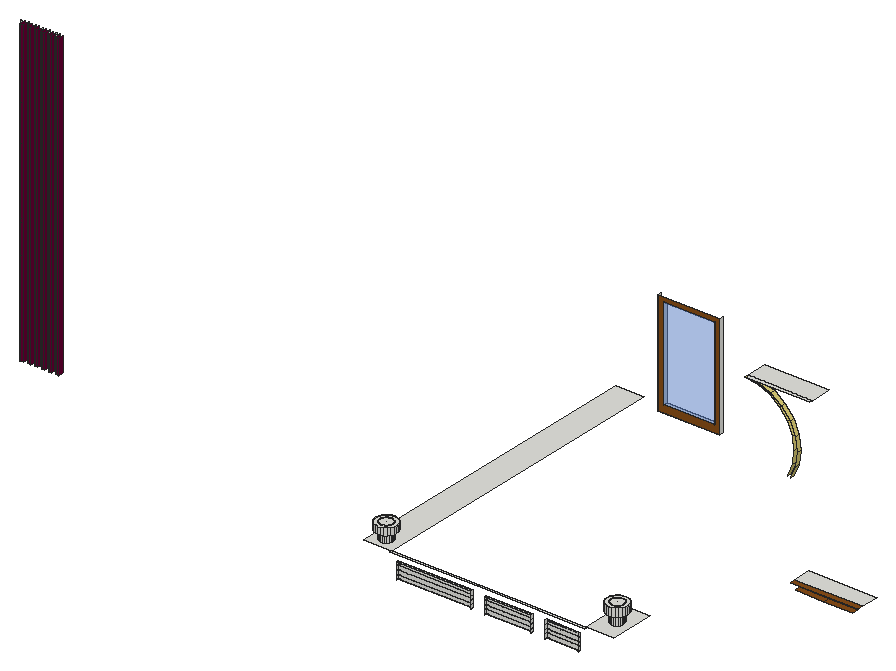
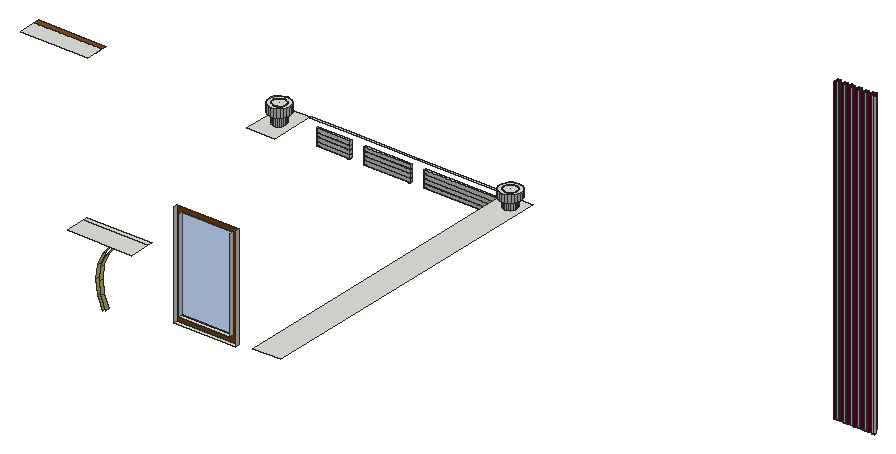
# SketchUp Ruby script. Lengths in inches.
U = 1.inch
M = Sketchup.active_model
def pt(a) = Geom::Point3d.new(a.map { |v| v * U })
def face(e, loops, mat)
  f = e.add_face(loops[0].map { |a| pt(a) })
  loops[1..].each { |l| e.add_face(l.map { |a| pt(a) }).erase! }
  f.material = f.back_material = mat if mat
  f
end
# faces: each face lists its corners as indices into pts; further lists are holes
def faces(e, pts, list, mat = nil) = list.each { |f| face(e, (f[0].is_a?(Array) ? f : [f]).map { |l| l.map { |i| pts[i] } }, mat) }
# xy, xz, yz: faces in a plane at the given z, y or x. An outline is a flat list of corners, or four numbers for a rectangle; further outlines are holes
def ring(l) = l.size == 4 ? [[l[0], l[1]], [l[2], l[1]], [l[2], l[3]], [l[0], l[3]]] : l.each_slice(2).to_a
def flat(e, list, mat, &to3) = list.each { |f| face(e, (f[0].is_a?(Array) ? f : [f]).map { |l| ring(l).map { |u, v| to3.(u, v) } }, mat) }
def xy(e, z, list, mat = nil) = flat(e, list, mat) { |x, y| [x, y, z] }
def xz(e, y, list, mat = nil) = flat(e, list, mat) { |x, z| [x, y, z] }
def yz(e, x, list, mat = nil) = flat(e, list, mat) { |y, z| [x, y, z] }
def lines(e, pts, list) = list.each { |a, b| e.add_line(pt(pts[a]), pt(pts[b])) }
# prism: a flat outline (further loops are holes) pulled along v
def prism(e, loops, v, mat = nil)
  f = face(e, loops, mat); d = Geom::Vector3d.new(v.map { |x| x * U })
  f.pushpull(f.normal.samedirection?(d) ? d.length : -d.length)
end
def box(e, o, s, mat = nil) = prism(e, [[o, [o[0] + s[0], o[1], o[2]], [o[0] + s[0], o[1] + s[1], o[2]], [o[0], o[1] + s[1], o[2]]]], [0, 0, s[2]], mat)
def at(x, y, z, deg = 0) = Geom::Transformation.translation(pt([x, y, z])) * Geom::Transformation.rotation(ORIGIN, Z_AXIS, deg.degrees)
def axes(o, x, y, z) = Geom::Transformation.new([*x, 0, *y, 0, *z, 0, *pt(o).to_a, 1])
def part(name) = M.definitions.add(name)
# library, detail: a bought-in or finely detailed component or shape, given as its bounding box
def library(name, o, s) = part(name).tap { |d| box(d.entities, o, s) }
def detail(e, o, s) = box(e.add_group.entities, o, s)
def put(e, d, t, mat = nil) = e.add_instance(d, t).tap { |i| i.material = mat if mat }
def group(e, t, mat = nil) = e.add_group.tap { |g| g.transformation = t; g.material = mat if mat }.entities
root = M.entities
M.materials.add("Teddy_SkinShadow ").color = [134, 77, 23]
M.materials.add("[Color L16]").color = [102, 0, 51]
M.materials.add("[Translucent Glass Blue]").color = [100, 149, 237]
M.materials["[Translucent Glass Blue]"].alpha = 0.5
M.materials.add("[Wood Board Cork]").color = [215, 201, 115]
xy(root,49.297,[[880.196,111.916,881.943,112.729],[883.778,111.916,885.525,112.729],[887.36,111.916,889.107,112.729],[869.45,112.041,871.197,112.729],[873.032,112.041,874.779,112.729],
  [876.614,112.041,878.361,112.729]])
xy(root,49.297,[[871.241,109.541,872.988,112.729],[881.987,109.854,883.734,112.729],[885.569,109.854,887.316,112.729],[889.151,109.854,890.942,112.729],[874.823,109.979,876.57,112.729],
  [878.405,109.979,880.152,112.729]],"[Color L16]")
xy(root,56.441,[[1147.452,64.973,1171.711,65.973],[1178.83,64.973,1196.125,65.973]])
xy(root,56.645,[[1101.817,64.973,1140.537,65.973]])
xy(root,57.564,[[1107.504,227.266,1139.629,229.266]])
xy(root,60,[[1098.461,64.973,1143.893,65.973],[1143.893,64.973,1175.271,65.973],[1175.271,64.973,1199.684,65.973],[[1084.247,65.973,1098.461,229.266],[1090.628,69,1089.738,69.117,1088.909,69.461,1088.197,70.007,1087.651,70.719,1087.308,71.548,1087.19,72.4375,1087.308,73.327,1087.651,74.156,1088.197,74.868,1088.909,75.414,1089.738,75.758,1090.628,75.875,1091.518,75.758,1092.347,75.414,1093.059,74.868,1093.605,74.156,1093.948,73.327,1094.065,72.4375,1093.948,71.548,1093.605,70.719,1093.059,70.007,1092.347,69.461,1091.518,69.117]]])
xy(root,60.1875,[[[1199.684,65.973,1213.899,88.973],[1206.602,73.728,1205.713,73.845,1204.883,74.189,1204.172,74.735,1203.625,75.447,1203.282,76.276,1203.165,77.166,1203.282,78.055,1203.625,78.884,1204.172,79.596,1204.883,80.143,1205.713,80.486,1206.602,80.603,1207.492,80.486,1208.321,80.143,1209.033,79.596,1209.579,78.884,1209.923,78.055,1210.04,77.166,1209.923,76.276,1209.579,75.447,1209.033,74.735,1208.321,74.189,1207.492,73.845]]])
xy(root,61.264,[[1110.481,227.266,1136.918,229.266]])
xy(root,64.5,[[[1090.628,66.975,1089.214,67.161,1087.897,67.707,1086.765,68.575,1085.897,69.706,1085.352,71.024,1085.165,72.4375,1085.352,73.851,1085.897,75.169,1086.765,76.3,1087.897,77.168,1089.214,77.714,1090.628,77.9,1092.042,77.714,1093.359,77.168,1094.491,76.3,1095.359,75.169,1095.904,73.851,1096.091,72.4375,1095.904,71.024,1095.359,69.706,1094.491,68.575,1093.359,67.707,1092.042,67.161],[1090.628,69,1091.518,69.117,1092.347,69.461,1093.059,70.007,1093.605,70.719,1093.948,71.548,1094.065,72.4375,1093.948,73.327,1093.605,74.156,1093.059,74.868,1092.347,75.414,1091.518,75.758,1090.628,75.875,1089.738,75.758,1088.909,75.414,1088.197,74.868,1087.651,74.156,1087.308,73.327,1087.19,72.4375,1087.308,71.548,1087.651,70.719,1088.197,70.007,1088.909,69.461,1089.738,69.117]]])
xy(root,65.375,[[[1206.602,71.703,1205.188,71.889,1203.871,72.435,1202.74,73.303,1201.871,74.434,1201.326,75.752,1201.14,77.166,1201.326,78.579,1201.871,79.897,1202.74,81.028,1203.871,81.896,1205.188,82.442,1206.602,82.628,1208.016,82.442,1209.333,81.896,1210.465,81.028,1211.333,79.897,1211.879,78.579,1212.065,77.166,1211.879,75.752,1211.333,74.434,1210.465,73.303,1209.333,72.435,1208.016,71.889],[1206.602,73.728,1207.492,73.845,1208.321,74.189,1209.033,74.735,1209.579,75.447,1209.923,76.276,1210.04,77.166,1209.923,78.055,1209.579,78.884,1209.033,79.596,1208.321,80.143,1207.492,80.486,1206.602,80.603,1205.713,80.486,1204.883,80.143,1204.172,79.596,1203.625,78.884,1203.282,78.055,1203.165,77.166,1203.282,76.276,1203.625,75.447,1204.172,74.735,1204.883,74.189,1205.713,73.845]]])
xy(root,68.125,[[[1090.628,66.975,1092.042,67.161,1093.359,67.707,1094.491,68.575,1095.359,69.706,1095.904,71.024,1096.091,72.4375,1095.904,73.851,1095.359,75.169,1094.491,76.3,1093.359,77.168,1092.042,77.714,1090.628,77.9,1089.214,77.714,1087.897,77.168,1086.765,76.3,1085.897,75.169,1085.352,73.851,1085.165,72.4375,1085.352,71.024,1085.897,69.706,1086.765,68.575,1087.897,67.707,1089.214,67.161],[1090.628,69,1089.738,69.117,1088.909,69.461,1088.197,70.007,1087.651,70.719,1087.308,71.548,1087.19,72.4375,1087.308,73.327,1087.651,74.156,1088.197,74.868,1088.909,75.414,1089.738,75.758,1090.628,75.875,1091.518,75.758,1092.347,75.414,1093.059,74.868,1093.605,74.156,1093.948,73.327,1094.065,72.4375,1093.948,71.548,1093.605,70.719,1093.059,70.007,1092.347,69.461,1091.518,69.117]],[1090.628,69,1091.518,69.117,1092.347,69.461,1093.059,70.007,1093.605,70.719,1093.948,71.548,1094.065,72.4375,1093.948,73.327,1093.605,74.156,1093.059,74.868,1092.347,75.414,1091.518,75.758,1090.628,75.875,1089.738,75.758,1088.909,75.414,1088.197,74.868,1087.651,74.156,1087.308,73.327,1087.19,72.4375,1087.308,71.548,1087.651,70.719,1088.197,70.007,1088.909,69.461,1089.738,69.117]])
xy(root,69.5,[[[1206.602,71.703,1208.016,71.889,1209.333,72.435,1210.465,73.303,1211.333,74.434,1211.879,75.752,1212.065,77.166,1211.879,78.579,1211.333,79.897,1210.465,81.028,1209.333,81.896,1208.016,82.442,1206.602,82.628,1205.188,82.442,1203.871,81.896,1202.74,81.028,1201.871,79.897,1201.326,78.579,1201.14,77.166,1201.326,75.752,1201.871,74.434,1202.74,73.303,1203.871,72.435,1205.188,71.889],[1206.602,73.728,1205.713,73.845,1204.883,74.189,1204.172,74.735,1203.625,75.447,1203.282,76.276,1203.165,77.166,1203.282,78.055,1203.625,78.884,1204.172,79.596,1204.883,80.143,1205.713,80.486,1206.602,80.603,1207.492,80.486,1208.321,80.143,1209.033,79.596,1209.579,78.884,1209.923,78.055,1210.04,77.166,1209.923,76.276,1209.579,75.447,1209.033,74.735,1208.321,74.189,1207.492,73.845]],[1206.602,73.728,1207.492,73.845,1208.321,74.189,1209.033,74.735,1209.579,75.447,1209.923,76.276,1210.04,77.166,1209.923,78.055,1209.579,78.884,1209.033,79.596,1208.321,80.143,1207.492,80.486,1206.602,80.603,1205.713,80.486,1204.883,80.143,1204.172,79.596,1203.625,78.884,1203.282,78.055,1203.165,77.166,1203.282,76.276,1203.625,75.447,1204.172,74.735,1204.883,74.189,1205.713,73.845]])
xy(root,84.352,[[1273.474,108.973,1288.316,111.973],[1288.316,108.973,1303.158,111.973]],"Teddy_SkinShadow ")
xy(root,86.936,[[1270.891,111.973,1305.742,120.973]])
xy(root,86.936,[[1270.891,108.973,1305.742,111.973]],"Teddy_SkinShadow ")
xy(root,88.919,[[1152.795,227.266,1186.043,229.266],[1152.795,229.266,1186.043,240.054]])
xz(root,65.973,[[1147.452,47.974,1171.711,47.993],[1178.83,47.979,1196.125,47.981],[1178.83,47.981,1196.125,50.095],[1147.452,47.993,1171.711,50.086],[1101.817,48.104,1140.537,48.121],
  [1101.817,48.121,1140.537,50.235],[1147.452,50.086,1171.711,50.105],[1178.83,50.095,1196.125,50.097],[1178.83,50.097,1196.125,52.21],[1147.452,50.105,1171.711,52.198],
  [1101.817,50.235,1140.537,50.252],[1101.817,50.252,1140.537,52.366],[1147.452,52.198,1171.711,52.217],[1178.83,52.21,1196.125,52.212],[1178.83,52.212,1196.125,54.325],
  [1147.452,52.217,1171.711,54.31],[1101.817,52.366,1140.537,52.383],[1101.817,52.383,1140.537,54.497],[1147.452,54.31,1171.711,54.329],[1178.83,54.325,1186.173,54.327],
  [1186.173,54.325,1196.125,54.327],[1178.83,54.327,1196.125,56.441],[1147.452,54.329,1171.711,56.441],[1101.817,54.497,1140.537,54.514],[1101.817,54.514,1140.537,56.645]])
xz(root,109.541,[[871.241,49.297,872.988,205.751]],"[Color L16]")
xz(root,109.854,[[881.987,49.297,883.734,205.751],[885.569,49.297,887.316,205.751],[889.151,49.297,890.942,205.751]],"[Color L16]")
xz(root,109.979,[[874.823,49.297,876.57,205.751],[878.405,49.297,880.152,205.751]],"[Color L16]")
xz(root,111.916,[[880.196,49.297,881.943,205.751],[883.778,49.297,885.525,205.751],[887.36,49.297,889.107,205.751]])
xz(root,112.041,[[869.45,49.297,871.197,205.751],[873.032,49.297,874.779,205.751],[876.614,49.297,878.361,205.751]])
xz(root,112.729,[[871.197,49.297,871.241,205.751],[872.988,49.297,873.032,205.751],[874.779,49.297,874.823,205.751],[876.57,49.297,876.614,205.751],[878.361,49.297,878.405,205.751],
  [880.152,49.297,880.196,205.751],[881.943,49.297,881.987,205.751],[883.734,49.297,883.778,205.751],[885.525,49.297,885.569,205.751],[887.316,49.297,887.36,205.751],
  [889.107,49.297,889.151,205.751]])
xz(root,227.266,[[[1107.504,57.564,1139.629,111.314],[1110.481,61.264,1136.918,109.014]]],"Teddy_SkinShadow ")
xz(root,227.266,[[1110.481,61.264,1136.918,109.014]],"[Translucent Glass Blue]")
yz(root,871.197,[[112.041,49.297,112.729,205.751]])
yz(root,871.241,[[109.541,49.297,112.729,205.751]],"[Color L16]")
yz(root,872.988,[[109.541,49.297,112.729,205.751]],"[Color L16]")
yz(root,873.032,[[112.041,49.297,112.729,205.751]])
yz(root,874.779,[[112.041,49.297,112.729,205.751]])
yz(root,874.823,[[109.979,49.297,112.729,205.751]],"[Color L16]")
yz(root,876.57,[[109.979,49.297,112.729,205.751]],"[Color L16]")
yz(root,876.614,[[112.041,49.297,112.729,205.751]])
yz(root,878.361,[[112.041,49.297,112.729,205.751]])
yz(root,878.405,[[109.979,49.297,112.729,205.751]],"[Color L16]")
yz(root,880.152,[[109.979,49.297,112.729,205.751]],"[Color L16]")
yz(root,880.196,[[111.916,49.297,112.729,205.751]])
yz(root,881.943,[[111.916,49.297,112.729,205.751]])
yz(root,881.987,[[109.854,49.297,112.729,205.751]],"[Color L16]")
yz(root,883.734,[[109.854,49.297,112.729,205.751]],"[Color L16]")
yz(root,883.778,[[111.916,49.297,112.729,205.751]])
yz(root,885.525,[[111.916,49.297,112.729,205.751]])
yz(root,885.569,[[109.854,49.297,112.729,205.751]],"[Color L16]")
yz(root,887.316,[[109.854,49.297,112.729,205.751]],"[Color L16]")
yz(root,887.36,[[111.916,49.297,112.729,205.751]])
yz(root,889.107,[[111.916,49.297,112.729,205.751]])
yz(root,889.151,[[109.854,49.297,112.729,205.751]],"[Color L16]")
yz(root,890.942,[[109.854,49.297,112.729,205.751]],"[Color L16]")
yz(root,1101.817,[[64.973,48.104,65.973,48.121],[64.973,48.121,65.973,50.235],[64.973,50.235,65.973,50.252],[64.973,50.252,65.973,52.366],[64.973,52.366,65.973,52.383],
  [64.973,52.383,65.973,54.497],[64.973,54.497,65.973,54.514],[64.973,54.514,65.973,56.645]])
yz(root,1107.504,[[227.266,57.564,229.266,111.314]])
yz(root,1110.481,[[227.266,61.264,229.266,109.014]])
yz(root,1136.918,[[227.266,61.264,229.266,109.014]])
yz(root,1139.629,[[227.266,57.564,229.266,111.314]])
yz(root,1140.537,[[64.973,48.104,65.973,48.121],[64.973,48.121,65.973,50.235],[64.973,50.235,65.973,50.252],[64.973,50.252,65.973,52.366],[64.973,52.366,65.973,52.383],
  [64.973,52.383,65.973,54.497],[64.973,54.497,65.973,54.514],[64.973,54.514,65.973,56.645]])
yz(root,1147.452,[[64.973,47.974,65.973,47.993],[64.973,47.993,65.973,50.086],[64.973,50.086,65.973,50.105],[64.973,50.105,65.973,52.198],[64.973,52.198,65.973,52.217],
  [64.973,52.217,65.973,54.31],[64.973,54.31,65.973,54.329],[64.973,54.329,65.973,56.441]])
yz(root,1171.711,[[64.973,47.974,65.973,47.993],[64.973,47.993,65.973,50.086],[64.973,50.086,65.973,50.105],[64.973,50.105,65.973,52.198],[64.973,52.198,65.973,52.217],
  [64.973,52.217,65.973,54.31],[64.973,54.31,65.973,54.329],[64.973,54.329,65.973,56.441]])
yz(root,1178.83,[[64.973,47.979,65.973,47.981],[64.973,47.981,65.973,50.095],[64.973,50.095,65.973,50.097],[64.973,50.097,65.973,52.21],[64.973,52.21,65.973,52.212],
  [64.973,52.212,65.973,54.325],[64.973,54.325,65.973,54.327],[64.973,54.327,65.973,56.441]])
yz(root,1196.125,[[64.973,47.979,65.973,47.981],[64.973,47.981,65.973,50.095],[64.973,50.095,65.973,50.097],[64.973,50.097,65.973,52.21],[64.973,52.21,65.973,52.212],
  [64.973,52.212,65.973,54.325],[64.973,54.325,65.973,54.327],[64.973,54.327,65.973,56.441]])
p = [[1179.097,229.266,56.737],[1176.326,229.266,50.38],[1176.326,227.266,50.38],[1179.097,227.266,56.737],[1174.716,229.266,50.951],[1177.245,229.266,57.056],
  [1177.245,227.266,57.056],[1174.716,227.266,50.951],[1180.045,229.266,63.607],[1180.045,227.266,63.607],[1178.107,229.266,63.607],[1178.107,227.266,63.607],
  [1089.738,69.117,60],[1090.628,69,60],[1090.628,69,64.5],[1089.738,69.117,64.5],[1091.518,69.117,60],[1091.518,69.117,64.5],
  [1088.909,69.461,60],[1088.909,69.461,64.5],[1092.347,69.461,60],[1092.347,69.461,64.5],[1088.197,70.007,60],[1088.197,70.007,64.5],
  [1093.059,70.007,60],[1093.059,70.007,64.5],[1087.651,70.719,60],[1087.651,70.719,64.5],[1093.605,70.719,60],[1093.605,70.719,64.5],
  [1087.308,71.548,60],[1087.308,71.548,64.5],[1093.948,71.548,60],[1093.948,71.548,64.5],[1087.19,72.4375,60],[1087.19,72.4375,64.5],
  [1094.065,72.4375,60],[1094.065,72.4375,64.5],[1087.308,73.327,60],[1087.308,73.327,64.5],[1093.948,73.327,60],[1093.948,73.327,64.5],
  [1087.651,74.156,60],[1087.651,74.156,64.5],[1093.605,74.156,60],[1093.605,74.156,64.5],[1088.197,74.868,60],[1088.197,74.868,64.5],
  [1093.059,74.868,60],[1093.059,74.868,64.5],[1088.909,75.414,60],[1088.909,75.414,64.5],[1092.347,75.414,60],[1092.347,75.414,64.5],
  [1089.738,75.758,60],[1089.738,75.758,64.5],[1091.518,75.758,60],[1091.518,75.758,64.5],[1090.628,75.875,60],[1090.628,75.875,64.5],
  [1205.713,73.845,60.1875],[1206.602,73.728,60.1875],[1206.602,73.728,65.375],[1205.713,73.845,65.375],[1207.492,73.845,60.1875],[1207.492,73.845,65.375],
  [1204.883,74.189,60.1875],[1204.883,74.189,65.375],[1208.321,74.189,60.1875],[1208.321,74.189,65.375],[1204.172,74.735,60.1875],[1204.172,74.735,65.375],
  [1209.033,74.735,60.1875],[1209.033,74.735,65.375],[1203.625,75.447,60.1875],[1203.625,75.447,65.375],[1209.579,75.447,60.1875],[1209.579,75.447,65.375],
  [1203.282,76.276,60.1875],[1203.282,76.276,65.375],[1209.923,76.276,60.1875],[1209.923,76.276,65.375],[1203.165,77.166,60.1875],[1203.165,77.166,65.375],
  [1210.04,77.166,60.1875],[1210.04,77.166,65.375],[1203.282,78.055,60.1875],[1203.282,78.055,65.375],[1209.923,78.055,60.1875],[1209.923,78.055,65.375],
  [1203.625,78.884,60.1875],[1203.625,78.884,65.375],[1209.579,78.884,60.1875],[1209.579,78.884,65.375],[1204.172,79.596,60.1875],[1204.172,79.596,65.375],
  [1209.033,79.596,60.1875],[1209.033,79.596,65.375],[1204.883,80.143,60.1875],[1204.883,80.143,65.375],[1208.321,80.143,60.1875],[1208.321,80.143,65.375],
  [1205.713,80.486,60.1875],[1205.713,80.486,65.375],[1207.492,80.486,60.1875],[1207.492,80.486,65.375],[1206.602,80.603,60.1875],[1206.602,80.603,65.375],
  [1177.245,229.266,70.158],[1177.245,227.266,70.158],[1179.097,229.266,70.477],[1179.097,227.266,70.477],[1089.214,67.161,64.5],[1090.628,66.975,64.5],
  [1090.628,66.975,68.125],[1089.214,67.161,68.125],[1092.042,67.161,64.5],[1092.042,67.161,68.125],[1087.897,67.707,64.5],[1087.897,67.707,68.125],
  [1093.359,67.707,64.5],[1093.359,67.707,68.125],[1086.765,68.575,64.5],[1086.765,68.575,68.125],[1094.491,68.575,64.5],[1094.491,68.575,68.125],
  [1085.897,69.706,64.5],[1085.897,69.706,68.125],[1095.359,69.706,64.5],[1095.359,69.706,68.125],[1089.738,69.117,68.125],[1090.628,69,68.125],
  [1091.518,69.117,68.125],[1088.909,69.461,68.125],[1092.347,69.461,68.125],[1088.197,70.007,68.125],[1093.059,70.007,68.125],[1085.352,71.024,64.5],
  [1085.352,71.024,68.125],[1095.904,71.024,64.5],[1095.904,71.024,68.125],[1087.651,70.719,68.125],[1093.605,70.719,68.125],[1087.308,71.548,68.125],
  [1093.948,71.548,68.125],[1085.165,72.4375,64.5],[1085.165,72.4375,68.125],[1096.091,72.4375,64.5],[1096.091,72.4375,68.125],[1087.19,72.4375,68.125],
  [1094.065,72.4375,68.125],[1085.352,73.851,64.5],[1085.352,73.851,68.125],[1087.308,73.327,68.125],[1093.948,73.327,68.125],[1095.904,73.851,64.5],
  [1095.904,73.851,68.125],[1087.651,74.156,68.125],[1093.605,74.156,68.125],[1085.897,75.169,64.5],[1085.897,75.169,68.125],[1095.359,75.169,64.5],
  [1095.359,75.169,68.125],[1088.197,74.868,68.125],[1093.059,74.868,68.125],[1088.909,75.414,68.125],[1092.347,75.414,68.125],[1086.765,76.3,64.5],
  [1086.765,76.3,68.125],[1094.491,76.3,64.5],[1094.491,76.3,68.125],[1089.738,75.758,68.125],[1091.518,75.758,68.125],[1090.628,75.875,68.125],
  [1087.897,77.168,64.5],[1087.897,77.168,68.125],[1093.359,77.168,64.5],[1093.359,77.168,68.125],[1089.214,77.714,64.5],[1089.214,77.714,68.125],
  [1092.042,77.714,64.5],[1092.042,77.714,68.125],[1090.628,77.9,64.5],[1090.628,77.9,68.125],[1205.188,71.889,65.375],[1206.602,71.703,65.375],
  [1206.602,71.703,69.5],[1205.188,71.889,69.5],[1208.016,71.889,65.375],[1208.016,71.889,69.5],[1203.871,72.435,65.375],[1203.871,72.435,69.5],
  [1209.333,72.435,65.375],[1209.333,72.435,69.5],[1202.74,73.303,65.375],[1202.74,73.303,69.5],[1210.465,73.303,65.375],[1210.465,73.303,69.5],
  [1201.871,74.434,65.375],[1201.871,74.434,69.5],[1211.333,74.434,65.375],[1211.333,74.434,69.5],[1205.713,73.845,69.5],[1206.602,73.728,69.5],
  [1207.492,73.845,69.5],[1204.883,74.189,69.5],[1208.321,74.189,69.5],[1204.172,74.735,69.5],[1209.033,74.735,69.5],[1201.326,75.752,65.375],
  [1201.326,75.752,69.5],[1211.879,75.752,65.375],[1211.879,75.752,69.5],[1203.625,75.447,69.5],[1209.579,75.447,69.5],[1203.282,76.276,69.5],
  [1209.923,76.276,69.5],[1201.14,77.166,65.375],[1201.14,77.166,69.5],[1212.065,77.166,65.375],[1212.065,77.166,69.5],[1203.165,77.166,69.5],
  [1210.04,77.166,69.5],[1201.326,78.579,65.375],[1201.326,78.579,69.5],[1203.282,78.055,69.5],[1209.923,78.055,69.5],[1211.879,78.579,65.375],
  [1211.879,78.579,69.5],[1203.625,78.884,69.5],[1209.579,78.884,69.5],[1201.871,79.897,65.375],[1201.871,79.897,69.5],[1211.333,79.897,65.375],
  [1211.333,79.897,69.5],[1204.172,79.596,69.5],[1209.033,79.596,69.5],[1204.883,80.143,69.5],[1208.321,80.143,69.5],[1202.74,81.028,65.375],
  [1202.74,81.028,69.5],[1210.465,81.028,65.375],[1210.465,81.028,69.5],[1205.713,80.486,69.5],[1207.492,80.486,69.5],[1206.602,80.603,69.5],
  [1203.871,81.896,65.375],[1203.871,81.896,69.5],[1209.333,81.896,65.375],[1209.333,81.896,69.5],[1205.188,82.442,65.375],[1205.188,82.442,69.5],
  [1208.016,82.442,65.375],[1208.016,82.442,69.5],[1206.602,82.628,65.375],[1206.602,82.628,69.5],[1174.716,229.266,76.263],[1174.716,227.266,76.263],
  [1176.326,229.266,76.834],[1176.326,227.266,76.834],[1170.693,229.266,81.506],[1170.693,227.266,81.506],[1171.937,229.266,82.203],[1171.937,227.266,82.203],
  [1165.451,229.266,85.528],[1165.451,227.266,85.528],[1166.259,229.266,86.185],[1166.259,227.266,86.185],[1159.346,229.266,88.057],[1159.346,227.266,88.057],
  [1159.715,229.266,88.48],[1159.715,227.266,88.48],[1152.795,229.266,88.919],[1152.795,227.266,88.919],[1186.173,65.973,54.31],[1186.173,65.973,54.325],
  [1206.602,77.166,65.375],[1206.602,77.166,69.5],[1090.419,72.396,64.5],[1090.419,72.396,68.125]]
faces(root,p,[[0,1,2,3],[4,5,6,7],[8,0,3,9],[5,10,11,6],[10,108,109,11],[110,8,9,111],[108,256,257,109],[258,110,111,259],
  [256,260,261,257],[262,258,259,263],[260,264,265,261],[266,262,263,267],[264,268,269,265],[270,266,267,271],[268,272,273,269],[272,270,271,273]],"[Wood Board Cork]")
faces(root,p,[[12,13,14,15],[13,16,17,14],[18,12,15,19],[16,20,21,17],[22,18,19,23],[20,24,25,21],[26,22,23,27],[24,28,29,25],
  [30,26,27,31],[28,32,33,29],[34,30,31,35],[32,36,37,33],[38,34,35,39],[36,40,41,37],[42,38,39,43],[40,44,45,41],
  [46,42,43,47],[44,48,49,45],[50,46,47,51],[48,52,53,49],[54,50,51,55],[52,56,57,53],[58,54,55,59],[56,58,59,57],
  [60,61,62,63],[61,64,65,62],[66,60,63,67],[64,68,69,65],[70,66,67,71],[68,72,73,69],[74,70,71,75],[72,76,77,73],
  [78,74,75,79],[76,80,81,77],[82,78,79,83],[80,84,85,81],[86,82,83,87],[84,88,89,85],[90,86,87,91],[88,92,93,89],
  [94,90,91,95],[92,96,97,93],[98,94,95,99],[96,100,101,97],[102,98,99,103],[100,104,105,101],[106,102,103,107],[104,106,107,105],
  [112,113,114,115],[113,116,117,114],[118,112,115,119],[116,120,121,117],[122,118,119,123],[120,124,125,121],[126,122,123,127],[124,128,129,125],
  [14,15,130,131],[17,14,131,132],[15,19,133,130],[21,17,132,134],[19,23,135,133],[25,21,134,136],[137,126,127,138],[128,139,140,129],
  [23,27,141,135],[29,25,136,142],[27,31,143,141],[33,29,142,144],[145,137,138,146],[139,147,148,140],[31,35,149,143],[37,33,144,150],
  [151,145,146,152],[35,39,153,149],[41,37,150,154],[147,155,156,148],[39,43,157,153],[45,41,154,158],[159,151,152,160],[155,161,162,156],
  [43,47,163,157],[49,45,158,164],[47,51,165,163],[53,49,164,166],[167,159,160,168],[161,169,170,162],[51,55,171,165],[57,53,166,172],
  [55,59,173,171],[59,57,172,173],[174,167,168,175],[169,176,177,170],[178,174,175,179],[176,180,181,177],[182,178,179,183],[180,182,183,181],
  [184,185,186,187],[185,188,189,186],[190,184,187,191],[188,192,193,189],[194,190,191,195],[192,196,197,193],[198,194,195,199],[196,200,201,197],
  [62,63,202,203],[65,62,203,204],[63,67,205,202],[69,65,204,206],[67,71,207,205],[73,69,206,208],[209,198,199,210],[200,211,212,201],
  [71,75,213,207],[77,73,208,214],[75,79,215,213],[81,77,214,216],[217,209,210,218],[211,219,220,212],[79,83,221,215],[85,81,216,222],
  [223,217,218,224],[83,87,225,221],[89,85,222,226],[219,227,228,220],[87,91,229,225],[93,89,226,230],[231,223,224,232],[227,233,234,228],
  [91,95,235,229],[97,93,230,236],[95,99,237,235],[101,97,236,238],[239,231,232,240],[233,241,242,234],[99,103,243,237],[105,101,238,244],
  [103,107,245,243],[107,105,244,245],[246,239,240,247],[241,248,249,242],[250,246,247,251],[248,252,253,249],[254,250,251,255],[252,254,255,253]])
lines(root,p,[[274,275],[276,277],[278,279]])
